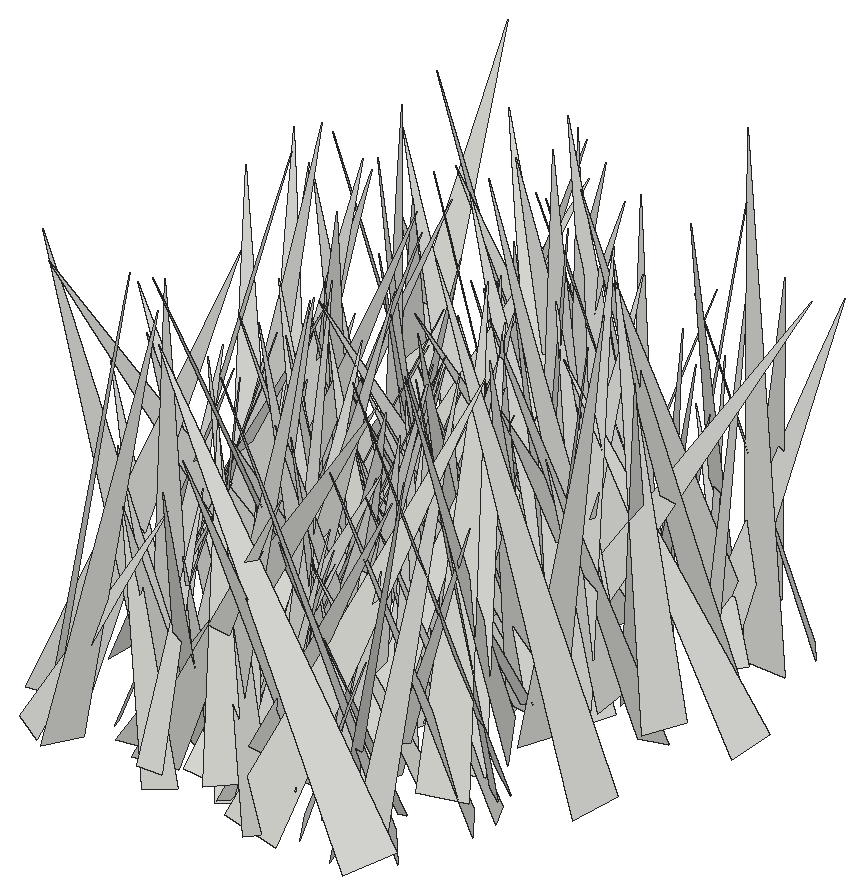
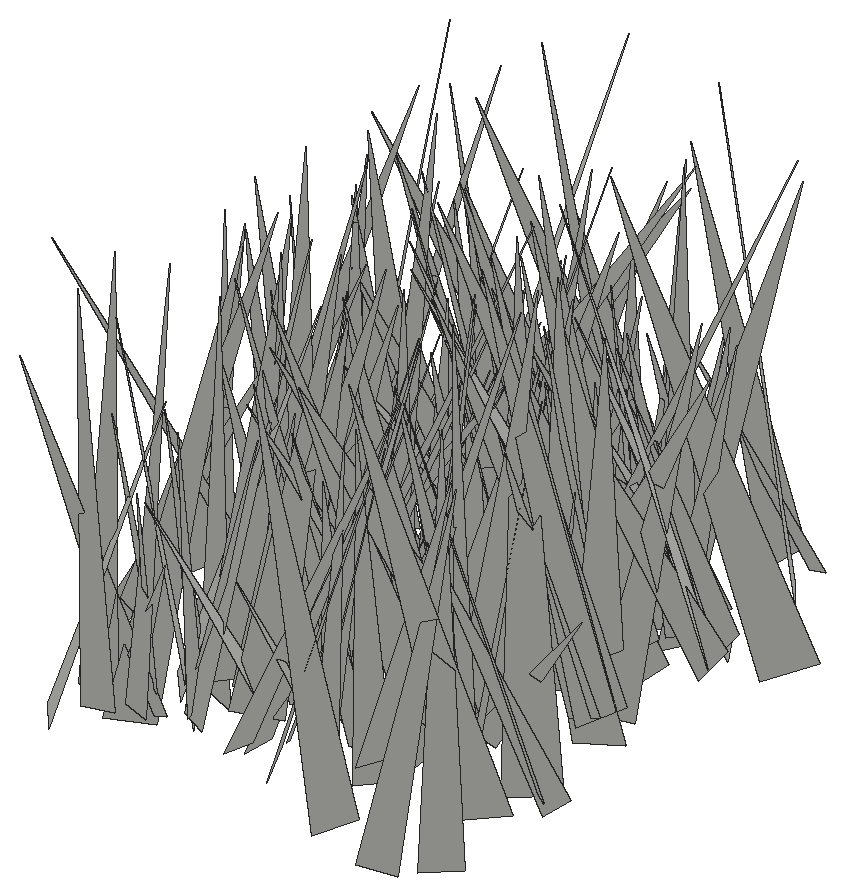
# SketchUp Ruby script. Lengths in inches.
U = 1.inch
M = Sketchup.active_model
def pt(a) = Geom::Point3d.new(a.map { |v| v * U })
def face(e, loops, mat)
  f = e.add_face(loops[0].map { |a| pt(a) })
  loops[1..].each { |l| e.add_face(l.map { |a| pt(a) }).erase! }
  f.material = f.back_material = mat if mat
  f
end
# faces: each face lists its corners as indices into pts; further lists are holes
def faces(e, pts, list, mat = nil) = list.each { |f| face(e, (f[0].is_a?(Array) ? f : [f]).map { |l| l.map { |i| pts[i] } }, mat) }
# xy, xz, yz: faces in a plane at the given z, y or x. An outline is a flat list of corners, or four numbers for a rectangle; further outlines are holes
def ring(l) = l.size == 4 ? [[l[0], l[1]], [l[2], l[1]], [l[2], l[3]], [l[0], l[3]]] : l.each_slice(2).to_a
def flat(e, list, mat, &to3) = list.each { |f| face(e, (f[0].is_a?(Array) ? f : [f]).map { |l| ring(l).map { |u, v| to3.(u, v) } }, mat) }
def xy(e, z, list, mat = nil) = flat(e, list, mat) { |x, y| [x, y, z] }
def xz(e, y, list, mat = nil) = flat(e, list, mat) { |x, z| [x, y, z] }
def yz(e, x, list, mat = nil) = flat(e, list, mat) { |y, z| [x, y, z] }
def lines(e, pts, list) = list.each { |a, b| e.add_line(pt(pts[a]), pt(pts[b])) }
# prism: a flat outline (further loops are holes) pulled along v
def prism(e, loops, v, mat = nil)
  f = face(e, loops, mat); d = Geom::Vector3d.new(v.map { |x| x * U })
  f.pushpull(f.normal.samedirection?(d) ? d.length : -d.length)
end
def box(e, o, s, mat = nil) = prism(e, [[o, [o[0] + s[0], o[1], o[2]], [o[0] + s[0], o[1] + s[1], o[2]], [o[0], o[1] + s[1], o[2]]]], [0, 0, s[2]], mat)
def at(x, y, z, deg = 0) = Geom::Transformation.translation(pt([x, y, z])) * Geom::Transformation.rotation(ORIGIN, Z_AXIS, deg.degrees)
def axes(o, x, y, z) = Geom::Transformation.new([*x, 0, *y, 0, *z, 0, *pt(o).to_a, 1])
def part(name) = M.definitions.add(name)
# library, detail: a bought-in or finely detailed component or shape, given as its bounding box
def library(name, o, s) = part(name).tap { |d| box(d.entities, o, s) }
def detail(e, o, s) = box(e.add_group.entities, o, s)
def put(e, d, t, mat = nil) = e.add_instance(d, t).tap { |i| i.material = mat if mat }
def group(e, t, mat = nil) = e.add_group.tap { |g| g.transformation = t; g.material = mat if mat }.entities
root = M.entities
c1 = part("fur_instance\#9")
p = [[0.8125,0,1.79],[0.67,-0.02,1.48],[0,-0.11,0],[0,0.11,0]]
faces(c1.entities,p,[[0,1,2,3]])
put(root,c1,axes([75.14,127.23,-28.22],[5.23311,-3.59302,0.50013],[-3.53385,-5.24745,-0.7222],[-0.81967,-0.31597,6.30664]))
put(root,c1,axes([77.73,116.96,-28.22],[-5.00326,5.02156,1.24961],[5.08502,5.09325,-0.10752],[0.95924,-0.80806,7.08781]))
put(root,c1,axes([76.61,128.3,-28.22],[1.62052,-5.44249,0.65001],[-5.43307,-1.68456,-0.55967],[-0.72449,0.45919,5.65098]))
put(root,c1,axes([76.89,117.4,-28.22],[2.93992,-5.13493,1.13143],[-5.01799,-3.12719,-1.15379],[-1.5708,0.37938,5.8034]))
put(root,c1,axes([78.92,120.61,-28.22],[-1.66623,3.3763,0.05798],[2.90925,1.40249,1.93607],[-1.71436,-0.9015,3.22914]))
put(root,c1,axes([74.32,123.78,-27.1],[4.41432,4.17138,0.78555],[4.1779,-4.06951,-1.86761],[0.75011,-1.88212,5.77916]))
put(root,c1,axes([74.86,122.39,-28.22],[4.12414,-1.44643,0.07491],[-1.4095,-3.95608,1.21201],[0.33327,1.1677,4.19901]))
put(root,c1,axes([76.14,124.13,-28.22],[-3.17908,7.18759,1.82609],[7.05927,3.54175,-1.65087],[2.27218,-0.9472,7.68392]))
put(root,c1,axes([78.04,113.14,-28.22],[-4.97411,1.9133,1.24146],[2.05101,5.05519,0.42681],[0.99764,-0.85328,5.31228]))
put(root,c1,axes([78.9375,112,-27.1],[-0.03383,-6.90938,2.82252],[-7.12958,-0.80509,-2.05628],[-2.20801,2.70547,6.5964]))
put(root,c1,axes([75.71,113.625,-27.1],[4.89085,0.64493,0.58721],[0.56841,-4.89366,0.64042],[-0.66156,0.56328,4.89144]))
put(root,c1,axes([74.62,112.25,-28.22],[5.54256,-5.39998,2.31392],[-5.86744,-4.92827,2.55329],[0.29519,3.43313,7.30483]))
put(root,c1,axes([75.87,114.34,-27.1],[6.07013,4.91373,1.22638],[4.90353,-6.18107,0.495],[-1.26656,-0.38061,7.79399]))
put(root,c1,axes([79.24,125.07,-27.1],[-5.48361,2.04542,0.49712],[2.0602,5.49974,0.09665],[0.43181,-0.2646,5.85187]))
put(root,c1,axes([76.24,119.43,-27.1],[-0.49271,4.25835,1.65602],[4.30491,0.99075,-1.26683],[1.53091,-1.41548,4.0953]))
put(root,c1,axes([75.3,114.83,-27.1],[5.97099,-0.01983,0.33196],[-0.11666,-5.7151,1.75709],[-0.31141,1.76085,5.70664]))
put(root,c1,axes([79,117.98,-27.1],[-7.67561,-3.02253,0.64542],[-2.50236,7.09168,3.4516],[1.81396,-3.00659,7.49247]))
put(root,c1,axes([80.64,114.66,-28.22],[-3.29072,5.65648,0.59206],[5.32719,2.82602,2.60955],[-1.99181,-1.7869,6.00123]))
put(root,c1,axes([78.19,116.21,-27.1],[2.36714,6.37429,1.14743],[6.22522,-2.57637,1.46983],[-1.78738,-0.5313,6.63886]))
put(root,c1,axes([77.01,113.96,-27.1],[-2.42701,4.03219,1.90827],[4.11447,2.86278,-0.81615],[1.72373,-1.15601,4.63496]))
put(root,c1,axes([76.87,112.09,-28.22],[4.59925,2.87418,0.36346],[2.61006,-4.40682,1.82035],[-1.25721,1.36572,5.10885]))
put(root,c1,axes([75.94,114.3125,-27.1],[3.19259,1.80159,0.09548],[1.75198,-3.04965,-1.03811],[0.43061,-0.9494,3.51578]))
put(root,c1,axes([75.89,119.11,-27.1],[6.31096,-2.97385,1.65761],[-3.28181,-6.24286,1.29466],[-0.9062,1.89806,6.85536]))
put(root,c1,axes([76.12,110.15,-27.1],[6.04593,4.4435,2.18806],[4.86244,-5.98205,-1.28733],[-0.94282,-2.35709,7.39194]))
put(root,c1,axes([76.24,118.78,-28.22],[-0.74897,7.24815,2.93985],[7.55595,1.43371,-1.60981],[2.0214,-2.6736,7.1067]))
put(root,c1,axes([78.82,116.89,-28.22],[-4.81371,6.17541,1.55135],[6.27572,4.93015,-0.15223],[1.07597,-1.1279,7.82843]))
put(root,c1,axes([75.84,122.27,-28.22],[5.44226,-5.9088,0.26751],[-5.91243,-5.44486,0.01623],[-0.16928,0.20777,8.03317]))
put(root,c1,axes([77.51,115.67,-27.1],[-6.57541,3.25527,2.97746],[2.73361,7.20101,-1.83599],[3.46258,0.49673,7.10365]))
put(root,c1,axes([77.93,122.11,-27.1],[-3.99319,-2.60087,1.40659],[-2.16034,4.18012,1.59628],[2.0189,-0.6713,4.49021]))
put(root,c1,axes([76.4,108.77,-27.1],[1.55212,3.88569,0.28277],[3.69063,-1.36892,-1.44671],[1.24813,-0.78428,3.92616]))
put(root,c1,axes([78.78,121.625,-27.1],[2.86323,5.98862,2.41998],[6.20716,-3.28322,0.78076],[-1.78634,-1.80966,6.59182]))
put(root,c1,axes([77.07,117.84,-27.1],[3.70766,-2.56946,0.56874],[-2.62102,-3.69364,0.39947],[-0.23628,0.65362,4.49325]))
put(root,c1,axes([78.86,120.99,-27.1],[-5.74569,2.33772,2.68731],[2.89131,6.03979,0.92776],[2.08013,-1.9379,6.13328]))
put(root,c1,axes([78.16,112.89,-27.1],[0.12589,-6.48138,2.39431],[-6.90548,-0.03647,0.26437],[0.23531,2.39734,6.47721]))
put(root,c1,axes([79.63,116.57,-28.22],[-4.02809,-0.22088,0.67447],[-0.39433,3.92835,-1.06856],[0.59008,1.11738,3.89005]))
put(root,c1,axes([77.59,108.78,-27.1],[6.54484,-1.1484,2.12677],[-1.53141,-6.71985,1.08414],[-1.86996,1.48383,6.55579]))
put(root,c1,axes([78.17,111.73,-27.1],[4.5765,3.32185,0.66717],[3.07667,-4.544,1.52],[-1.41913,0.86116,5.4469]))
put(root,c1,axes([80.59,122.84,-27.1],[-4.6315,-5.30606,1.24554],[-5.44783,4.55599,-0.84886],[0.16366,1.49838,6.99175]))
put(root,c1,axes([80.09,109.92,-28.22],[-1.43576,4.62376,1.24523],[4.74317,1.1948,1.0324],[-0.65727,-1.47798,4.73019]))
put(root,c1,axes([79.01,112.52,-28.22],[-3.93498,0.71077,2.15609],[1.47172,4.08376,1.33974],[1.72857,-1.85895,3.76754]))
put(root,c1,axes([78.09,114.38,-28.22],[-4.16703,-2.76107,2.92288],[-2.78486,5.0182,0.77013],[2.90022,0.85149,4.93909]))
put(root,c1,axes([77.52,123.15,-28.22],[3.73133,2.74864,1.27928],[3.02044,-3.19509,-1.94493],[0.26177,-2.31318,4.20655]))
put(root,c1,axes([78.04,116.5,-28.22],[6.99612,0.8962,1.32294],[0.53893,-6.91662,1.83548],[-1.5043,1.69005,6.81028]))
put(root,c1,axes([80.41,117.08,-28.22],[2.01081,5.29668,2.07869],[5.40677,-2.46554,1.0522],[-1.77275,-1.51176,5.56697]))
put(root,c1,axes([78.77,121.27,-27.1],[5.20805,0.62891,1.21236],[0.54515,-5.33937,0.42794],[-1.25226,0.29119,5.2284]))
put(root,c1,axes([80.96,120.82,-28.22],[-6.68963,-2.36331,2.10659],[-2.62997,6.88987,-0.62215],[1.76244,1.31094,7.06748]))
put(root,c1,axes([77.53,115.21,-28.22],[7.81962,-2.04899,1.63917],[-2.46618,-7.49875,2.3913],[-0.8962,2.75717,7.72182]))
put(root,c1,axes([79.55,118.46,-28.22],[3.89032,1.8987,0.46131],[1.51623,-3.58179,1.95558],[-1.23244,1.58688,3.86204]))
put(root,c1,axes([79.625,122.46,-27.1],[-2.94569,-5.43055,1.36405],[-5.282,3.20651,1.35919],[1.85796,0.50597,6.02666]))
put(root,c1,axes([79.81,126.62,-27.1],[-0.67343,-4.75938,1.30258],[-4.88536,0.82798,0.49956],[0.69398,1.21023,4.78075]))
put(root,c1,axes([80.6,120.42,-27.1],[1.77342,-4.13167,0.71101],[-4.001,-1.89854,-1.053],[-1.2523,0.21471,4.37115]))
put(root,c1,axes([82.64,125.36,-28.22],[-7.3033,-3.33888,1.09507],[-3.45877,7.27632,-0.88176],[0.61989,1.26191,7.98178]))
put(root,c1,axes([80.0625,112.42,-28.22],[0.55845,-3.67703,0.59896],[-3.72525,-0.55803,0.04757],[-0.0423,0.59936,3.71889]))
put(root,c1,axes([81.74,115.86,-28.22],[-2.9661,5.6248,1.68099],[5.86235,2.73802,1.18234],[-0.31135,-2.03143,6.24805]))
put(root,c1,axes([80.48,109,-27.1],[0.12612,4.07155,0.3622],[4.08216,-0.1442,0.19951],[-0.2114,-0.35539,4.06861]))
put(root,c1,axes([79.77,124.48,-28.22],[3.7544,-3.60472,1.46029],[-3.77286,-3.86843,0.15082],[-0.94444,1.12393,5.20257]))
put(root,c1,axes([80.79,126.08,-27.1],[-3.85431,-2.63258,1.04926],[-2.43046,3.98156,1.06172],[1.4575,-0.32233,4.54521]))
put(root,c1,axes([78.37,120.73,-27.1],[-2.47927,6.31853,1.78834],[5.49074,3.04318,-3.14001],[3.60191,-0.28983,6.01756]))
put(root,c1,axes([79.02,127.13,-28.22],[6.16664,-2.56617,1.31423],[-2.70082,-6.22755,0.51287],[-1.00896,0.98602,6.65955]))
put(root,c1,axes([79.29,114.13,-28.22],[6.54433,-2.87567,1.841],[-3.10892,-6.66403,0.64215],[-1.41189,1.3447,7.11937]))
put(root,c1,axes([79.33,114.77,-28.22],[3.69637,0.13401,0.11411],[0.12786,-3.69317,0.19555],[-0.12096,0.19138,3.69362]))
put(root,c1,axes([82.76,126.82,-27.1],[-6.27523,-0.24227,0.55286],[-0.1392,6.19931,1.13667],[0.58735,-1.11924,6.17618]))
put(root,c1,axes([79.1,116.72,-28.22],[2.01974,-4.62687,0.27657],[-4.52399,-1.90214,1.21619],[1.00891,0.73329,4.89981]))
put(root,c1,axes([81.07,117.35,-28.22],[-5.69321,-2.11736,2.09192],[-1.78965,6.04293,1.24584],[2.37833,-0.52131,5.94506]))
put(root,c1,axes([79.36,112.42,-28.22],[-1.30326,-6.4856,0.41929],[-6.05179,1.36694,2.33336],[2.36951,-0.07596,6.19006]))
put(root,c1,axes([82.1,110.5,-28.22],[-1.23415,4.06964,0.18802],[4.01431,1.18128,0.78126],[-0.69473,-0.40381,4.18028]))
put(root,c1,axes([81.25,125.07,-27.1],[0.8668,-4.44855,1.11397],[-4.54098,-0.99091,-0.42373],[-0.6404,1.00517,4.51236]))
put(root,c1,axes([79.57,121.95,-28.22],[7.57177,-0.43303,1.80554],[-0.88332,-7.50835,1.90355],[-1.63317,2.05334,7.34137]))
put(root,c1,axes([82.95,122.9375,-27.1],[-4.95008,-4.07189,1.35786],[-4.2827,4.82407,-1.14641],[0.2873,1.75371,6.30629]))
put(root,c1,axes([83.84,109.58,-28.22],[-6.70082,0.16595,0.10129],[0.12128,6.29761,-2.29436],[0.15195,2.29157,6.29797]))
put(root,c1,axes([80.6,111.15,-28.22],[-1.68385,4.77561,0.18208],[4.53538,1.65768,-1.53538],[1.50664,0.34725,4.82539]))
put(root,c1,axes([81.94,111.48,-28.22],[-3.57041,1.71359,0.7726],[1.61509,3.64514,-0.62093],[0.96166,0.24019,3.91135]))
put(root,c1,axes([79.71,114.17,-27.1],[5.6659,3.07924,0.02777],[3.03508,-5.59401,1.03936],[-0.52039,0.90013,6.36426]))
put(root,c1,axes([81.0625,124.34,-28.22],[3.38601,2.0667,0.33408],[1.88033,-3.28152,1.24252],[-0.92044,0.89903,3.76728]))
put(root,c1,axes([83.63,124.83,-28.22],[-5.15429,0.32159,0.0951],[0.32057,5.15491,-0.05731],[0.09848,0.05128,5.164]))
put(root,c1,axes([82.58,109.59,-27.1],[-4.08375,3.22336,1.0157],[3.24667,4.18417,-0.22495],[0.93853,-0.4488,5.19774]))
put(root,c1,axes([81.89,125.66,-27.1],[-4.9139,-3.74374,0.55427],[-3.15126,4.55055,2.79845],[2.0958,-1.9355,5.50733]))
put(root,c1,axes([79.12,110.96,-28.22],[3.81653,-4.78014,0.36891],[-4.62204,-3.54318,1.90641],[1.2738,1.46558,5.81217]))
put(root,c1,axes([82.8,122.19,-28.22],[-3.67286,3.55796,0.5072],[3.52102,3.70767,-0.51167],[0.72023,0.01818,5.08794]))
put(root,c1,axes([82.17,117.22,-28.22],[3.62515,-5.36286,0.15908],[-5.03579,-3.46731,-2.13211],[-1.85105,-1.06996,6.11196]))
put(root,c1,axes([80.52,112.37,-28.22],[3.29309,2.39527,0.08068],[2.3726,-3.23886,-0.68467],[0.3385,-0.60058,4.0141]))
put(root,c1,axes([82.92,116.33,-28.22],[3.41803,-2.18502,2.15563],[-1.95303,-4.03718,-0.99543],[-2.36786,0.1758,3.93273]))
put(root,c1,axes([83.11,113.98,-28.22],[-6.84332,-0.22544,2.15666],[-0.013,7.14388,0.70553],[2.16837,-0.66867,6.81058]))
put(root,c1,axes([82.75,110.85,-28.22],[-5.5806,3.5391,0.90465],[3.04631,5.42049,-2.4135],[2.01583,1.60617,6.15169]))
put(root,c1,axes([81.15,113,-28.22],[7.05742,-1.09775,2.22467],[-1.64487,-7.09246,1.71837],[-1.85705,2.1103,6.93249]))
put(root,c1,axes([84.02,110.39,-27.1],[2.20032,6.76237,0.49836],[6.15454,-2.21163,2.83722],[-2.84601,0.44546,6.52083]))
put(root,c1,axes([80.43,116.63,-28.22],[3.57739,2.98141,0.96801],[3.07785,-3.06266,-1.94177],[0.59384,-2.08684,4.23274]))
put(root,c1,axes([80.62,114.6,-27.1],[4.47916,2.33614,0.04477],[2.33654,-4.47877,-0.05982],[-0.01203,-0.07375,5.05142]))
put(root,c1,axes([78.38,111.47,-28.22],[6.17977,-5.38552,0.13557],[-5.06059,-5.73249,2.95646],[1.84733,2.31224,7.64543]))
put(root,c1,axes([84.18,114.64,-27.1],[-6.24569,-2.79636,0.92417],[-2.76847,6.31368,0.39421],[1.00464,0.01396,6.83176]))
put(root,c1,axes([83.37,120.02,-27.1],[-4.08154,-1.42978,0.42723],[-1.12455,3.76494,1.85644],[0.98091,-1.633,3.906]))
put(root,c1,axes([84.31,115.09,-28.22],[-2.33709,5.71521,1.48586],[5.84354,2.00796,1.46781],[-0.85111,-1.90732,5.99759]))
put(root,c1,axes([82.98,122.04,-28.22],[-2.39364,-3.13142,1.17859],[-3.27618,2.48779,-0.04385],[0.67935,0.9641,3.94124]))
put(root,c1,axes([81.83,120.13,-27.1],[5.28462,2.45266,0.54887],[2.09175,-5.00051,2.20534],[-1.39334,1.79538,5.39252]))
put(root,c1,axes([80.82,114.31,-27.1],[5.67742,2.27779,0.25934],[2.25803,-5.67581,0.41845],[-0.39608,0.29237,6.10297]))
put(root,c1,axes([84.24,121.15,-27.1],[-6.53247,-2.60599,0.49941],[-2.30056,6.22381,2.3844],[1.32211,-2.04617,6.61657]))
put(root,c1,axes([80.52,117.15,-28.22],[1.7793,-6.50243,0.4842],[-6.28195,-1.575,1.93351],[1.74732,0.95904,6.45825]))
put(root,c1,axes([81.21,111.09,-27.1],[-2.12698,-6.60371,3.80122],[-7.1046,3.14508,1.48842],[2.75369,3.0136,6.77625]))
put(root,c1,axes([82.15,111.3,-28.22],[3.75823,0.40452,0.85087],[0.18545,-3.74836,0.96295],[-0.9237,0.89332,3.65522]))
put(root,c1,axes([80.67,112.83,-27.1],[0.36945,4.73641,1.83647],[4.53767,0.52011,-2.25427],[2.28381,-1.79961,4.18191]))
put(root,c1,axes([83.32,113.58,-27.1],[-4.36965,-1.59831,1.51111],[-1.58231,4.61869,0.30967],[1.52785,0.21216,4.64247]))
put(root,c1,axes([87.43,111.375,-27.1],[-5.76145,-5.93812,0.42997],[-5.44241,5.01036,-3.73055],[-2.41379,2.87671,7.38502]))
put(root,c1,axes([83.51,125.05,-27.1],[3.66547,-5.8791,2.24711],[-5.89364,-4.11869,-1.16204],[-2.20868,1.23351,6.83002]))
put(root,c1,axes([85.71,121.38,-28.22],[-6.13421,5.52562,0.24546],[5.52788,6.11218,0.5523],[-0.18784,-0.57446,8.23747]))
put(root,c1,axes([81.66,119.64,-27.1],[4.65487,-3.05281,1.35089],[-3.29302,-4.57961,0.99778],[-0.54826,1.58741,5.47649]))
put(root,c1,axes([81.79,114.86,-27.1],[1.56073,-4.1385,0.9971],[-4.17951,-1.28812,1.1957],[0.80812,1.33073,4.25833]))
put(root,c1,axes([81.15,123.19,-28.22],[2.86437,6.58912,2.04567],[6.83224,-2.40073,-1.83379],[0.96006,-2.57407,6.94682]))
put(root,c1,axes([83.92,119.51,-28.22],[2.45384,5.3856,0.3895],[5.06414,-2.44383,1.88676],[-1.87372,0.44803,5.60947]))
put(root,c1,axes([83.02,111.01,-27.1],[1.48501,3.27806,0.44782],[3.28348,-1.52047,0.24164],[-0.40618,-0.30651,3.59062]))
put(root,c1,axes([84.82,119.79,-28.22],[-5.60277,-1.40853,0.55452],[-1.25772,5.51462,1.29985],[0.84237,-1.13469,5.62898]))
put(root,c1,axes([84.7,111.1875,-27.1],[-1.00098,-5.50903,0.83943],[-5.47181,0.81017,-1.20786],[-1.05515,1.02481,5.46739]))
put(root,c1,axes([83.875,118.45,-27.1],[-3.49973,-1.74713,0.54329],[-1.50598,3.41664,1.28623],[1.03907,-0.93268,3.69408]))
put(root,c1,axes([86.24,118.33,-27.1],[-2.89235,-4.23355,0.19447],[-3.82387,2.50545,-2.32964],[-1.82723,1.45817,4.56743]))
put(root,c1,axes([83.93,121.53,-28.22],[-4.28945,-4.51982,0.83876],[-4.25056,4.33652,1.63064],[1.75072,-0.54543,6.01408]))
put(root,c1,axes([82.28,114.51,-28.22],[4.17066,5.06918,1.33611],[5.23853,-4.09478,-0.81653],[-0.19883,-1.55319,6.51339]))
put(root,c1,axes([82.6,123.4,-27.1],[0.98375,-3.96673,0.69714],[-3.91068,-0.76919,1.14174],[0.96305,0.9285,3.92417]))
put(root,c1,axes([88.48,108.66,-27.1],[-3.77529,6.85051,0.02559],[5.94676,3.26269,3.89536],[-3.40091,-1.89957,6.78296]))
put(root,c1,axes([85.98,114.97,-27.1],[-4.15206,-1.52587,0.16301],[-1.50616,3.96212,-1.27574],[-0.29385,1.25209,4.2356]))
put(root,c1,axes([84.51,114.27,-27.1],[-3.56654,2.39752,0.7344],[2.22273,3.6139,-1.00345],[1.16058,0.44646,4.17868]))
put(root,c1,axes([84.79,115.62,-27.1],[-4.53937,1.16522,1.40638],[1.15678,4.75002,-0.2018],[1.41333,-0.14527,4.6822]))
put(root,c1,axes([83.35,118.79,-27.1],[1.74282,-4.6233,0.69197],[-4.67126,-1.6936,0.44965],[0.18179,0.80496,4.92038]))
put(root,c1,axes([83.8125,124.25,-27.1],[3.6245,2.89722,0.22495],[2.66528,-3.45765,1.58821],[-1.15791,1.11007,4.35987]))
put(root,c1,axes([84.66,123.93,-27.1],[-2.85824,2.70123,1.97363],[3.21945,2.92659,0.65696],[0.90938,-1.87078,3.87745]))
put(root,c1,axes([82.78,113.6875,-28.22],[3.79421,5.57197,1.64798],[5.81056,-3.63804,-1.07735],[0.00109,-1.96889,6.65448]))
put(root,c1,axes([85.58,125.24,-27.1],[-4.70558,-0.80345,0.83315],[-0.88013,4.74917,-0.39105],[0.7517,0.53106,4.75763]))
put(root,c1,axes([83.74,112.79,-28.22],[4.84887,3.21318,0.05137],[2.84684,-4.33809,2.62966],[-1.49084,2.16682,5.18854]))
put(root,c1,axes([84.68,126.45,-27.1],[-3.9391,-6.11846,0.96009],[-6.01065,4.05101,1.1555],[1.49311,0.1661,7.18449]))
put(root,c1,axes([86.24,125.11,-27.1],[-5.08924,-4.37631,0.84531],[-4.44671,5.07308,-0.50754],[0.30556,0.93743,6.69289]))
put(root,c1,axes([87.02,120.09,-28.22],[-7.32829,2.58062,0.59876],[2.60966,7.33524,0.32553],[0.45582,-0.50666,7.76257]))
put(root,c1,axes([83.85,123.17,-27.1],[3.80262,-6.94068,2.14426],[-7.19034,-3.9408,-0.00453],[-1.0344,1.87826,7.9141]))
put(root,c1,axes([85.44,123.95,-27.1],[-6.5147,3.53544,2.59254],[3.94464,6.75335,0.70282],[1.91322,-1.88542,7.3788]))
put(root,c1,axes([85.15,122.18,-28.22],[-3.37227,-0.8607,0.92289],[-0.91034,3.4828,-0.07828],[0.87397,0.30665,3.4795]))
put(root,c1,axes([82.16,110.76,-28.22],[5.56558,-2.4926,0.3103],[-2.49513,-5.39934,1.38077],[0.28926,1.38533,5.93988]))
put(root,c1,axes([86.06,120.88,-27.1],[-7.47088,0.3057,1.86762],[-0.12287,7.51123,-1.721],[1.88848,1.69808,7.27638]))
put(root,c1,axes([83.92,122.14,-28.22],[-0.35457,5.93898,1.63328],[6.05839,0.63143,-0.98081],[1.11129,-1.54746,5.86815]))
put(root,c1,axes([83,121.375,-28.22],[1.38948,-7.3294,0.52561],[-7.22169,-1.26322,1.47599],[1.35779,0.7818,7.31247]))
put(root,c1,axes([85.99,120.34,-28.22],[-5.98871,-2.33617,1.80164],[-2.60473,6.10133,-0.74665],[1.38529,1.37273,6.38474]))
put(root,c1,axes([83.57,119.47,-27.1],[-0.94018,-7.50089,0.47804],[-7.29693,1.02641,1.75419],[1.80188,0.24278,7.35324]))
put(root,c1,axes([83.75,114.03,-28.22],[4.94298,-3.20176,1.42299],[-3.34359,-5.04595,0.26096],[-1.0472,0.99819,5.88356]))
put(root,c1,axes([86.57,118.87,-27.1],[-4.85696,2.92878,0.85344],[3.03677,4.79447,0.82904],[0.29007,-1.15391,5.61075]))
put(root,c1,axes([84.18,121.24,-28.22],[5.33637,4.77614,2.80857],[5.34994,-5.45601,-0.88678],[-1.44141,-2.56842,7.10647]))
put(root,c1,axes([85.04,114.38,-27.1],[-2.3678,2.48019,1.72309],[2.76192,2.66404,-0.03926],[1.22155,-1.2159,3.42875]))
put(root,c1,axes([84.49,112.65,-28.22],[-1.93845,6.02083,0.54238],[5.77969,2.01278,-1.68701],[1.77192,0.02133,6.09606]))
put(root,c1,axes([86.71,113.28,-27.1],[-3.57731,-0.93265,0.01118],[-0.92223,3.54345,0.51048],[0.1395,-0.49118,3.66148]))
put(root,c1,axes([84.96,125.97,-27.1],[4.07501,0.67414,1.38281],[0.80205,-4.27202,-0.28088],[-1.31276,-0.5174,4.12083]))
put(root,c1,axes([87.2,111.44,-28.22],[-6.16047,-5.25921,0.96963],[-5.25018,6.22911,0.42963],[1.01736,0.29959,8.08864]))
put(root,c1,axes([85.42,123.29,-27.1],[4.02503,-3.95124,0.17731],[-3.62061,-3.78264,-2.10414],[-1.59215,-1.38705,5.23314]))
put(root,c1,axes([85.03,115.95,-27.1],[3.51726,-1.23078,1.44078],[-1.67757,-3.4351,1.16087],[-0.88116,1.62697,3.54095]))
put(root,c1,axes([85.13,111.43,-28.22],[-1.45732,3.49071,1.72371],[3.67662,1.83923,-0.61623],[1.28012,-1.30851,3.73217]))
put(root,c1,axes([86.39,123.36,-28.22],[1.78909,6.44129,2.50482],[6.73985,-2.19865,0.83993],[-1.52927,-2.15428,6.63216]))
put(root,c1,axes([83.51,109.62,-28.22],[-0.75445,7.6495,1.46212],[7.18414,1.25072,-2.83648],[3.00677,-1.06897,7.14412]))
put(root,c1,axes([87.99,120,-27.1],[-7.83982,-0.95667,1.33619],[-0.96404,7.9519,0.03699],[1.33088,0.12461,7.89789]))
put(root,c1,axes([85.69,119.78,-27.1],[4.582,2.26461,1.64468],[2.3704,-4.81752,0.02956],[-1.48816,-0.70087,5.111]))
put(root,c1,axes([84.92,121.6,-27.1],[1.46313,-3.34357,0.17988],[-3.25058,-1.37123,0.95187],[0.80348,0.54115,3.52337]))
put(root,c1,axes([86.77,119.59,-28.22],[-4.32916,0.66549,1.27706],[0.40908,4.44763,-0.93094],[1.38073,0.76884,4.27993]))
put(root,c1,axes([85.29,125.25,-27.1],[4.21688,0.53755,0.91963],[0.65776,-4.26755,-0.52159],[-0.83787,-0.64478,4.21888]))
put(root,c1,axes([84.51,110.66,-28.22],[3.70621,1.73352,0.50221],[1.78343,-3.34171,-1.62653],[0.27688,-1.67963,3.75439]))
put(root,c1,axes([87.31,120.32,-27.1],[1.60632,-4.77246,2.92285],[-5.28453,-2.29441,-0.84211],[-1.84207,2.42054,4.96463]))
put(root,c1,axes([85.41,119.52,-28.22],[0.50064,-7.21064,0.91051],[-7.21991,-0.3887,0.89157],[0.83387,0.96363,7.17281]))
put(root,c1,axes([88.29,114.5625,-28.22],[-4.47388,-2.50611,0.21033],[-2.51468,4.46372,-0.30343],[0.03476,0.36756,5.119]))
put(root,c1,axes([86.93,125.48,-27.1],[1.67627,3.15128,1.04901],[3.10636,-1.90337,0.75402],[-1.17538,-0.53615,3.48882]))
put(root,c1,axes([86.14,124.59,-28.22],[5.20843,4.28763,1.83578],[4.29945,-5.48037,0.60158],[-1.80791,-0.68076,6.71935]))
put(root,c1,axes([88.23,125.04,-28.22],[-0.98772,3.5916,0.11089],[3.35733,0.88143,1.35606],[-1.28071,-0.45933,3.46934]))
put(root,c1,axes([87.25,114.16,-27.1],[-2.49742,5.95651,1.04282],[6.02179,2.55284,-0.16018],[0.55273,-0.89868,6.45689]))
put(root,c1,axes([86.32,126.98,-27.1],[-2.86307,-5.78602,1.82095],[-5.78172,3.21211,1.11581],[1.83453,1.09334,6.35847]))
put(root,c1,axes([88,113.8,-28.22],[-4.87517,-3.87645,0.62854],[-3.83008,4.91477,0.6039],[0.86741,-0.08574,6.19915]))
put(root,c1,axes([89.01,120.41,-28.22],[-2.01567,-6.30283,1.43527],[-6.28052,1.55369,-1.99742],[-1.52993,1.92587,6.30864]))
put(root,c1,axes([87.1,119.07,-27.1],[-0.4945,6.57851,1.5324],[6.75453,0.47319,0.14829],[-0.03697,-1.53911,6.5954]))
put(root,c1,axes([85.92,112.71,-27.1],[4.29201,-0.29938,0.77765],[-0.39482,-4.32378,0.51456],[-0.73381,0.57535,4.27156]))
put(root,c1,axes([87.73,112.78,-27.1],[-1.40207,7.22786,1.13046],[7.31414,1.36087,0.37039],[-0.15287,-1.17973,7.35327]))
put(root,c1,axes([88.69,113.83,-27.1],[2.96491,4.33641,3.25393],[4.46173,-4.05854,1.34327],[-3.07985,-1.70497,5.07846]))
put(root,c1,axes([87.34,125.96,-28.22],[5.45366,-4.66647,1.60556],[-4.21255,-5.64853,-2.10822],[-2.57063,-0.64365,6.86103]))
put(root,c1,axes([88.41,114.5625,-27.1],[-4.17901,-5.88434,0.7845],[-5.89024,4.22956,0.34775],[0.73891,0.43633,7.20893]))
put(root,c1,axes([87.95,109.21,-27.1],[1.53889,6.65129,0.3221],[6.53467,-1.57198,1.24039],[-1.28121,-0.02868,6.71336]))
put(root,c1,axes([85.99,110.45,-28.22],[6.26752,1.77798,1.53658],[2.00319,-6.33057,-0.84565],[-1.22862,-1.25168,6.45971]))
put(root,c1,axes([89.69,122.7,-27.1],[-2.64388,-6.79077,2.11498],[-6.99476,2.07362,-2.08599],[-1.28885,2.67645,6.98236]))
put(root,c1,axes([86.55,118.54,-28.22],[6.67765,-1.57713,2.05629],[-1.75682,-6.93326,0.38749],[-1.90506,0.86558,6.85042]))
put(root,c1,axes([87.21,116.44,-27.1],[-6.01376,-4.74049,2.00405],[-3.98095,6.23797,2.80955],[3.26197,-1.12665,7.12348]))
put(root,c1,axes([88.76,123.14,-27.1],[2.37609,4.94692,0.8109],[4.47755,-2.49789,2.11838],[-2.25414,0.25283,5.06264]))
put(root,c1,axes([89.33,127.13,-28.22],[-4.41159,-3.54695,0.73212],[-3.61607,4.3782,-0.57829],[0.20221,0.91078,5.63104]))
put(root,c1,axes([84.14,121.13,-28.22],[3.56611,7.00423,0.23479],[6.50816,-3.2121,-3.02618],[2.59966,-1.56674,7.25387]))
put(root,c1,axes([88.86,125.48,-28.22],[1.25442,7.48082,2.76942],[7.81491,-1.71475,1.09211],[-1.59984,-2.51056,7.50623]))
put(root,c1,axes([86.875,122.43,-28.22],[6.59264,-0.88288,1.14982],[-0.53637,-6.4595,-1.88457],[-1.3468,-1.74924,6.37893]))
put(root,c1,axes([91.35,114.95,-27.1],[-8.2127,0.65784,0.53458],[0.66874,8.22786,0.14871],[0.52088,-0.19122,8.23766]))
put(root,c1,axes([87.22,127.53,-27.1],[-0.17668,-5.97479,1.5156],[-5.97573,0.53792,1.42395],[1.51188,1.4279,5.80532]))
put(root,c1,axes([90.06,119.6,-27.1],[-6.40273,2.01611,1.14645],[1.98655,6.50456,-0.34415],[1.19695,-0.01086,6.70383]))
put(root,c1,axes([91.3,121.82,-28.22],[-6.11827,1.22354,0.04324],[1.20265,5.96505,1.37981],[-0.22923,-1.36132,6.08493]))
put(root,c1,axes([87.13,125.36,-28.22],[0.44188,5.84269,1.52194],[5.83939,-0.02571,-1.59672],[1.53457,-1.58458,5.63763]))
